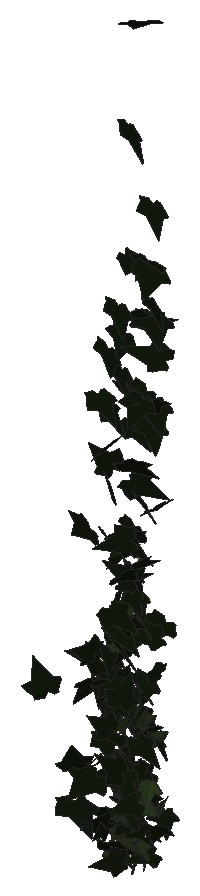
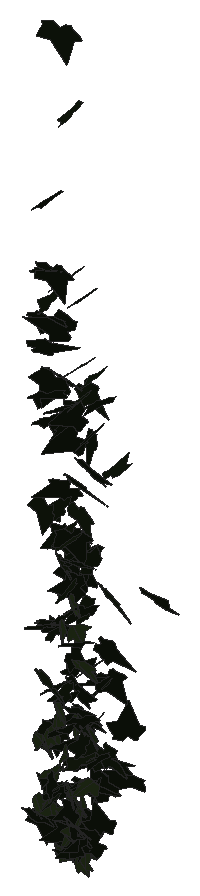
# SketchUp Ruby script. Lengths in inches.
U = 1.inch
M = Sketchup.active_model
def pt(a) = Geom::Point3d.new(a.map { |v| v * U })
def face(e, loops, mat)
  f = e.add_face(loops[0].map { |a| pt(a) })
  loops[1..].each { |l| e.add_face(l.map { |a| pt(a) }).erase! }
  f.material = f.back_material = mat if mat
  f
end
# faces: each face lists its corners as indices into pts; further lists are holes
def faces(e, pts, list, mat = nil) = list.each { |f| face(e, (f[0].is_a?(Array) ? f : [f]).map { |l| l.map { |i| pts[i] } }, mat) }
# xy, xz, yz: faces in a plane at the given z, y or x. An outline is a flat list of corners, or four numbers for a rectangle; further outlines are holes
def ring(l) = l.size == 4 ? [[l[0], l[1]], [l[2], l[1]], [l[2], l[3]], [l[0], l[3]]] : l.each_slice(2).to_a
def flat(e, list, mat, &to3) = list.each { |f| face(e, (f[0].is_a?(Array) ? f : [f]).map { |l| ring(l).map { |u, v| to3.(u, v) } }, mat) }
def xy(e, z, list, mat = nil) = flat(e, list, mat) { |x, y| [x, y, z] }
def xz(e, y, list, mat = nil) = flat(e, list, mat) { |x, z| [x, y, z] }
def yz(e, x, list, mat = nil) = flat(e, list, mat) { |y, z| [x, y, z] }
def lines(e, pts, list) = list.each { |a, b| e.add_line(pt(pts[a]), pt(pts[b])) }
# prism: a flat outline (further loops are holes) pulled along v
def prism(e, loops, v, mat = nil)
  f = face(e, loops, mat); d = Geom::Vector3d.new(v.map { |x| x * U })
  f.pushpull(f.normal.samedirection?(d) ? d.length : -d.length)
end
def box(e, o, s, mat = nil) = prism(e, [[o, [o[0] + s[0], o[1], o[2]], [o[0] + s[0], o[1] + s[1], o[2]], [o[0], o[1] + s[1], o[2]]]], [0, 0, s[2]], mat)
def at(x, y, z, deg = 0) = Geom::Transformation.translation(pt([x, y, z])) * Geom::Transformation.rotation(ORIGIN, Z_AXIS, deg.degrees)
def axes(o, x, y, z) = Geom::Transformation.new([*x, 0, *y, 0, *z, 0, *pt(o).to_a, 1])
def part(name) = M.definitions.add(name)
# library, detail: a bought-in or finely detailed component or shape, given as its bounding box
def library(name, o, s) = part(name).tap { |d| box(d.entities, o, s) }
def detail(e, o, s) = box(e.add_group.entities, o, s)
def put(e, d, t, mat = nil) = e.add_instance(d, t).tap { |i| i.material = mat if mat }
def group(e, t, mat = nil) = e.add_group.tap { |g| g.transformation = t; g.material = mat if mat }.entities
root = M.entities
M.materials.add("1026 AP 7946 SUNNY SIDE UP").color = [254, 231, 186]
M.materials.add("efeu1").color = [18, 25, 13]
M.materials.add("efeu2").color = [43, 57, 29]
c1 = part("ivyleaf_10")
p = [[0,0.5,-0.03],[-0.0625,2.02,-0.43],[-0.19,2.01,-0.46],[-0.54,1.05,-0.29],[-0.52,0.625,-0.18],[-0.83,0.76,-0.28],
  [-1.16,0.64,-0.33],[-1.15,0.33,-0.24],[-0.77,-0.39,0.02],[-0.3,-0.51,0.16],[0.04,-0.48,0.23],[-0.02,2.01,-0.4375],
  [-0.06,2.01,-0.43],[0.04,-0.49,0.23],[0.67,-0.49,0.14],[1.38,0.36,-0.2],[1.375,0.51,-0.24],[0.81,0.65,-0.19],
  [0.62,0.59,-0.15],[0.6,1.09,-0.28],[0.5,1.23,-0.31]]
faces(c1.entities,p,[[0,1,2,3,4,5,6,7,8,9,10],[11,12,0,13,14,15,16,17,18,19,20]],"efeu2")
c2 = part("ivyleaf_9")
p = [[1.54,2.16,1.25],[1.36,2.04,1.19],[-0.21,0.99,0.68],[-0.71,1.11,0.82],[-0.85,0.86,0.67],[-0.8,0.17,0.21],
  [-0.9,-0.01,0.1],[-0.67,-0.16,-0.02],[-0.08,-0.08,-0.05],[-0.03,-0.6,-0.4],[0.65,-0.88,-0.66],[0.83,-0.6,-0.49],
  [1.29,-0.42,-0.43],[1.8125,-0.07,-0.26],[1.21,0.44,0.15]]
faces(c2.entities,p,[[0,1,2,3,4,5,6,7,8,9,10,11,12,13,14]],"efeu1")
put(root,c1,axes([137.83,211.51,297.38],[0.4012,-0.28176,-0.05488],[-0.07373,0.02718,-0.39107],[0.44435,0.25891,-0.01534]),"1026 AP 7946 SUNNY SIDE UP")
put(root,c2,axes([137.54,211.69,314.56],[0.01331,-0.40991,0.19079],[0.02943,-0.18708,-0.42325],[0.70819,0.01547,0.014]),"1026 AP 7946 SUNNY SIDE UP")
put(root,c2,axes([138.35,209.95,300.61],[-0.17209,0.02371,-0.4585],[-0.6701,-0.14021,0.09942],[-0.2059,0.43649,0.05967]),"1026 AP 7946 SUNNY SIDE UP")
put(root,c2,axes([137.45,211.55,292.13],[0.51397,0.13779,0.20311],[0.29466,0.06056,-0.36476],[-0.23551,0.37648,-0.01311]),"1026 AP 7946 SUNNY SIDE UP")
put(root,c2,axes([138.01,210.06,299.29],[-0.00822,0.28996,-0.33221],[0.02756,-0.32374,-0.30055],[-0.68326,-0.01655,-0.00812]),"1026 AP 7946 SUNNY SIDE UP")
put(root,c2,axes([137.67,211.26,296],[-0.00138,-0.36582,-0.11151],[-0.01405,0.10615,-0.37614],[0.59879,0.00165,-0.00908]),"1026 AP 7946 SUNNY SIDE UP")
put(root,c1,axes([137.91,212.06,291.31],[-0.03657,-0.34127,0.1456],[-0.00683,-0.14329,-0.35319],[0.58194,-0.02313,0.005]),"1026 AP 7946 SUNNY SIDE UP")
put(root,c2,axes([137.6,211.53,311.9],[0.26933,-0.37215,-0.18863],[-0.11711,0.16496,-0.42108],[0.64008,0.18677,0.00233]),"1026 AP 7946 SUNNY SIDE UP")
put(root,c1,axes([138.09,211.77,291.07],[-0.4496,0.1913,-0.15349],[-0.17696,0.10123,0.35442],[0.3389,0.30664,-0.01857]),"1026 AP 7946 SUNNY SIDE UP")
put(root,c2,axes([137.67,211.29,297.84],[0.3313,-0.2889,-0.23528],[-0.14859,0.20996,-0.36483],[0.55803,0.22743,0.04254]),"1026 AP 7946 SUNNY SIDE UP")
put(root,c2,axes([138.39,210.875,309.48],[-0.09102,0.24213,0.41038],[-0.42897,0.30627,-0.23164],[-0.5921,-0.25911,0.10473]),"1026 AP 7946 SUNNY SIDE UP")
put(root,c1,axes([137.73,211.64,294.87],[-0.22919,-0.20056,-0.30427],[0.34422,0.20026,-0.25118],[0.44157,-0.2602,0.03788]),"1026 AP 7946 SUNNY SIDE UP")
put(root,c2,axes([138.15,210.05,295.625],[-0.32693,0.29532,-0.22341],[0.12696,-0.20824,-0.37025],[-0.56356,-0.21823,0.04619]),"1026 AP 7946 SUNNY SIDE UP")
put(root,c2,axes([137.67,210.85,292.39],[0.61428,-0.06207,-0.01055],[0.02521,0.03823,0.40561],[-0.09556,-0.38891,0.0392]),"1026 AP 7946 SUNNY SIDE UP")
put(root,c1,axes([138.18,211.67,300.53],[0.49868,-0.12912,-0.19854],[-0.30965,0.02036,-0.34911],[0.19098,0.37017,-0.04761]),"1026 AP 7946 SUNNY SIDE UP")
put(root,c2,axes([137.94,211.94,298.11],[-0.20399,-0.34986,-0.10126],[0.05213,0.09042,-0.38387],[0.56819,-0.1339,-0.00113]),"1026 AP 7946 SUNNY SIDE UP")
put(root,c2,axes([137.95,212.26,315.18],[-0.14688,-0.37961,0.20878],[-0.00701,-0.2087,-0.40181],[0.6782,-0.08437,0.04106]),"1026 AP 7946 SUNNY SIDE UP")
put(root,c2,axes([137.68,211.54,305.46],[0.1914,-0.26591,0.33434],[0.23774,-0.2891,-0.30273],[0.61737,0.19377,0.01293]),"1026 AP 7946 SUNNY SIDE UP")
put(root,c2,axes([137.72,212.07,296.91],[0.37537,-0.28468,0.14955],[0.10506,-0.13478,-0.38203],[0.49256,0.2457,-0.03249]),"1026 AP 7946 SUNNY SIDE UP")
put(root,c2,axes([138.34,209.76,294.98],[-0.6747,-0.20928,0.03821],[-0.02552,-0.05372,-0.49032],[0.33356,-0.42743,0.03977]),"1026 AP 7946 SUNNY SIDE UP")
put(root,c2,axes([138.07,208.66,295.9],[0.43434,0.21469,0.30903],[-0.40918,-0.15006,0.35808],[0.40892,-0.3782,0.03007]),"1026 AP 7946 SUNNY SIDE UP")
put(root,c2,axes([138.65,211.18,294.4],[-0.5417,0.0012,0.27766],[-0.42114,-0.05037,-0.35275],[0.04732,-0.43449,0.03909]),"1026 AP 7946 SUNNY SIDE UP")
put(root,c2,axes([137.9,210.63,312.9],[0.09758,-0.39034,-0.19905],[0.02644,0.19495,-0.40368],[0.6828,0.04824,0.04407]),"1026 AP 7946 SUNNY SIDE UP")
put(root,c2,axes([137.96,212.09,313.51],[0.08002,-0.41551,0.10142],[-0.00389,-0.1018,-0.43159],[0.67229,0.04887,-0.01457]),"1026 AP 7946 SUNNY SIDE UP")
put(root,c2,axes([138.04,210.51,298.89],[-0.02751,-0.31744,0.23075],[0.00706,-0.22617,-0.32854],[0.61249,-0.01165,0.01415]),"1026 AP 7946 SUNNY SIDE UP")
put(root,c1,axes([138.29,211.92,302.27],[-0.24082,-0.31947,0.17507],[0.06064,-0.19973,-0.34845],[0.5671,-0.11431,0.11161]),"1026 AP 7946 SUNNY SIDE UP")
put(root,c2,axes([138.09,211.24,300.18],[-0.05447,-0.38917,0.11404],[-0.00962,-0.11281,-0.40315],[0.6371,-0.03498,0.00366]),"1026 AP 7946 SUNNY SIDE UP")
put(root,c2,axes([138,208.9,293.96],[-0.29707,-0.26418,-0.36455],[0.39707,0.24915,-0.33046],[0.56735,-0.3127,0.0404]),"1026 AP 7946 SUNNY SIDE UP")
put(root,c2,axes([138.73,211.28,298.89],[-0.06949,0.10664,0.46598],[-0.3435,0.39558,-0.11591],[-0.64392,-0.22253,0.01154]),"1026 AP 7946 SUNNY SIDE UP")
put(root,c1,axes([138.32,211.61,293.21],[-0.3447,0.29579,0.03313],[-0.06057,0.00929,-0.37833],[-0.46362,-0.22113,0.0248]),"1026 AP 7946 SUNNY SIDE UP")
put(root,c2,axes([138.375,212.02,294.69],[-0.25939,-0.21116,0.2866],[-0.17091,-0.26272,-0.27221],[0.52349,-0.19041,0.05314]),"1026 AP 7946 SUNNY SIDE UP")
put(root,c2,axes([138.29,212.125,301.71],[-0.34152,-0.32796,0.04261],[0.07011,-0.08026,-0.39702],[0.51539,-0.2064,0.08224]),"1026 AP 7946 SUNNY SIDE UP")
put(root,c2,axes([138.76,206.01,300.99],[-0.71849,0.06801,-0.137],[-0.20114,0.04522,0.47549],[0.12232,0.47385,-0.02285]),"1026 AP 7946 SUNNY SIDE UP")
put(root,c2,axes([138.39,211,299.3125],[-0.33496,-0.33533,0.14859],[-0.07402,-0.14257,-0.40856],[0.57038,-0.21542,0.03424]),"1026 AP 7946 SUNNY SIDE UP")
put(root,c2,axes([137.96,212.05,312.84],[0.65535,-0.11657,0.09573],[0.12224,-0.06776,-0.444],[0.20077,0.42175,-0.04216]),"1026 AP 7946 SUNNY SIDE UP")
put(root,c2,axes([138.02,211.89,295.85],[0.05295,-0.43187,0.13889],[0.24199,-0.11857,-0.42388],[0.67019,0.07693,0.14208]),"1026 AP 7946 SUNNY SIDE UP")
put(root,c2,axes([138.52,211.8125,305.46],[-0.57268,-0.16871,-0.04043],[0.12797,-0.08835,-0.39703],[0.24004,-0.3554,0.11522]),"1026 AP 7946 SUNNY SIDE UP")
put(root,c2,axes([138.48,211.31,297.53],[-0.38477,0.14602,-0.29034],[0.34675,-0.17918,-0.29309],[-0.36058,-0.32813,0.02797]),"1026 AP 7946 SUNNY SIDE UP")
put(root,c2,axes([138.1,211.93,291.69],[0.50683,-0.17534,0.05451],[0.04919,-0.05485,-0.37681],[0.28421,0.32217,-0.03199]),"1026 AP 7946 SUNNY SIDE UP")
put(root,c2,axes([138.31,210.33,295.53],[-0.09367,0.39647,-0.18602],[-0.03098,0.18188,0.41403],[0.6858,0.06237,-0.00671]),"1026 AP 7946 SUNNY SIDE UP")
put(root,c2,axes([138.91,211.92,292.9375],[-0.36654,0.22115,0.20028],[-0.27084,0.09674,-0.32769],[-0.37391,-0.28686,0.04103]),"1026 AP 7946 SUNNY SIDE UP")
put(root,c1,axes([138.62,211.98,294.51],[0.20419,-0.30117,-0.21215],[-0.1395,0.18408,-0.33672],[0.5549,0.15711,-0.00659]),"1026 AP 7946 SUNNY SIDE UP")
put(root,c2,axes([138.01,211.98,291.92],[0.4199,-0.14774,0.26811],[0.33213,-0.15562,-0.31419],[0.33495,0.33951,-0.02456]),"1026 AP 7946 SUNNY SIDE UP")
put(root,c2,axes([138.6,211.48,291.7],[-0.40329,0.29124,-0.04141],[-0.02237,0.04317,0.39963],[0.46211,0.25626,-0.01679]),"1026 AP 7946 SUNNY SIDE UP")
put(root,c2,axes([138.82,211.33,297.99],[-0.61747,-0.07745,0.04565],[-0.05714,-0.04596,-0.41077],[0.12852,-0.39255,0.03667]),"1026 AP 7946 SUNNY SIDE UP")
put(root,c1,axes([138.42,211.7,292.39],[-0.36047,-0.24316,-0.20815],[0.27678,0.10712,-0.34026],[0.41127,-0.28521,0.04655]),"1026 AP 7946 SUNNY SIDE UP")
put(root,c1,axes([138.55,211.8,303.49],[0.21611,-0.34974,0.13106],[0.05423,-0.12518,-0.38763],[0.58375,0.14111,-0.01251]),"1026 AP 7946 SUNNY SIDE UP")
put(root,c1,axes([139.03,211.3,293.49],[-0.16669,0.09849,0.35885],[-0.55507,0.04967,-0.12505],[-0.12213,-0.36017,0.07858]),"1026 AP 7946 SUNNY SIDE UP")
put(root,c2,axes([138.52,211.76,293.34],[0.1528,0.1864,0.32703],[0.2826,0.26126,-0.21391],[-0.50352,0.2032,-0.02082]),"1026 AP 7946 SUNNY SIDE UP")
put(root,c1,axes([138.625,212.3,296.36],[-0.02972,0.25303,-0.30258],[-0.0139,-0.2957,-0.2623],[-0.61113,-0.00558,0.02068]),"1026 AP 7946 SUNNY SIDE UP")
put(root,c2,axes([138.95,211.88,291.33],[-0.53508,-0.12315,0.05816],[-0.06758,-0.04858,-0.37176],[0.20249,-0.34162,0.0296]),"1026 AP 7946 SUNNY SIDE UP")
put(root,c1,axes([138.63,210.82,291.07],[-0.3755,-0.21027,-0.17548],[0.28174,0.04534,-0.31841],[0.31729,-0.28911,0.07507]),"1026 AP 7946 SUNNY SIDE UP")
put(root,c2,axes([138.82,211.48,300.74],[-0.15976,0.14562,-0.38123],[0.29349,-0.32077,-0.1843],[-0.55353,-0.2121,0.01231]),"1026 AP 7946 SUNNY SIDE UP")
put(root,c2,axes([138.5,211.79,319.36],[0.35909,-0.33894,-0.22388],[-0.08184,0.22071,-0.41336],[0.62613,0.22324,0.07436]),"1026 AP 7946 SUNNY SIDE UP")
put(root,c2,axes([138.73,212.0625,297.45],[-0.17677,-0.36124,0.04195],[-0.00377,-0.04403,-0.38986],[0.57197,-0.11194,0.01039]),"1026 AP 7946 SUNNY SIDE UP")
put(root,c2,axes([139.03,211.24,306.33],[0.1522,0.33957,-0.27374],[-0.09624,-0.26075,-0.36513],[-0.67301,0.11408,-0.00969]),"1026 AP 7946 SUNNY SIDE UP")
put(root,c2,axes([138.33,211.85,292.28],[0.00097,-0.07821,-0.48898],[0.57512,0.3077,-0.04999],[0.49025,-0.36082,0.05961]),"1026 AP 7946 SUNNY SIDE UP")
put(root,c1,axes([138.89,210.75,293.28],[0.15458,-0.32954,-0.21242],[0.03113,0.21478,-0.34579],[0.60889,0.07268,0.07161]),"1026 AP 7946 SUNNY SIDE UP")
put(root,c2,axes([138.74,212.31,296.78],[-0.1279,-0.37344,0.00884],[0.00588,-0.01177,-0.39375],[0.58741,-0.0812,0.00587]),"1026 AP 7946 SUNNY SIDE UP")
put(root,c2,axes([138.58,212.09,304.07],[0.16065,-0.3766,0.15164],[0.04144,-0.1475,-0.40266],[0.63567,0.10479,-0.01207]),"1026 AP 7946 SUNNY SIDE UP")
put(root,c2,axes([138.6875,212.1,302.96],[0.05258,-0.42335,-0.05714],[-0.02251,0.05208,-0.43706],[0.6705,0.03495,-0.01019]),"1026 AP 7946 SUNNY SIDE UP")
put(root,c2,axes([138.75,211.93,306.28],[-0.1103,-0.3326,0.23208],[0.04421,-0.23407,-0.34547],[0.63178,-0.04169,0.0647]),"1026 AP 7946 SUNNY SIDE UP")
put(root,c1,axes([138.94,210.96,297.31],[-0.01767,-0.37872,-0.14308],[0.06137,0.13512,-0.38806],[0.63014,-0.02378,0.03378]),"1026 AP 7946 SUNNY SIDE UP")
put(root,c2,axes([138.68,211.22,303.88],[0.20812,0.15279,0.39844],[0.45912,0.25358,-0.20512],[-0.4638,0.31958,-0.02426]),"1026 AP 7946 SUNNY SIDE UP")
put(root,c2,axes([139.21,211.82,330.98],[0.22632,0.44363,-0.10633],[-0.23462,-0.05896,-0.46446],[-0.67764,0.16858,0.1253]),"1026 AP 7946 SUNNY SIDE UP")
put(root,c1,axes([138.85,211.43,291.28],[-0.46663,-0.16687,-0.15755],[0.26352,0.00526,-0.34304],[0.23773,-0.33338,0.07101]),"1026 AP 7946 SUNNY SIDE UP")
put(root,c1,axes([139.04,211.95,302.37],[0.35366,-0.31054,-0.10888],[0.0137,0.13171,-0.38524],[0.51472,0.20986,0.08507]),"1026 AP 7946 SUNNY SIDE UP")
put(root,c2,axes([138.86,211.55,292.92],[-0.05808,-0.37097,-0.08603],[0.04003,0.07919,-0.38319],[0.59585,-0.04148,0.01736]),"1026 AP 7946 SUNNY SIDE UP")
put(root,c2,axes([139.5,208.26,302.0625],[-0.37994,0.35783,0.17823],[-0.17097,0.13276,-0.44378],[-0.59969,-0.26456,0.0136]),"1026 AP 7946 SUNNY SIDE UP")
put(root,c2,axes([139.09,212.27,312.8125],[-0.35496,-0.32314,0.17721],[-0.05067,-0.18587,-0.4001],[0.57474,-0.21595,0.07417]),"1026 AP 7946 SUNNY SIDE UP")
put(root,c2,axes([138.82,209.08,292.97],[0.49659,0.29216,0.10893],[-0.15698,-0.04487,0.44158],[0.46172,-0.32948,0.03297]),"1026 AP 7946 SUNNY SIDE UP")
put(root,c2,axes([138.75,211.84,299.03],[0.43938,-0.27258,0.02814],[0.00719,-0.03657,-0.40167],[0.43095,0.27853,-0.02199]),"1026 AP 7946 SUNNY SIDE UP")
put(root,c2,axes([139.02,211.6,298.68],[-0.19779,-0.36412,0.05604],[-0.00849,-0.05784,-0.39695],[0.57932,-0.12516,0.01332]),"1026 AP 7946 SUNNY SIDE UP")
put(root,c2,axes([138.94,212.04,297.3],[0.19255,-0.27874,-0.26677],[-0.0578,0.26046,-0.30709],[0.59374,0.11575,0.05662]),"1026 AP 7946 SUNNY SIDE UP")
put(root,c2,axes([138.94,210.62,317.5625],[0.0218,-0.44722,0.06102],[0.00222,-0.06176,-0.46131],[0.70988,0.01393,-0.00043]),"1026 AP 7946 SUNNY SIDE UP")
put(root,c2,axes([139.16,208.3125,307.95],[-0.36413,-0.18579,0.38399],[-0.01767,-0.42453,-0.22704],[0.65611,-0.11454,0.20699]),"1026 AP 7946 SUNNY SIDE UP")
put(root,c2,axes([139.58,210.65,294.71],[-0.33883,-0.05141,0.36616],[-0.4782,-0.19495,-0.21996],[0.30117,-0.36737,0.06269]),"1026 AP 7946 SUNNY SIDE UP")
put(root,c2,axes([139.3,209.95,303.39],[-0.0023,-0.01127,0.48334],[0.22189,0.44753,0.01414],[-0.70391,0.14111,0.00288]),"1026 AP 7946 SUNNY SIDE UP")
put(root,c2,axes([139.27,212.32,294.35],[-0.28665,-0.19834,0.26709],[-0.07785,-0.27791,-0.25542],[0.50877,-0.15427,0.1114]),"1026 AP 7946 SUNNY SIDE UP")
put(root,c2,axes([139.46,211.98,319.32],[0.41668,0.11052,-0.36401],[-0.45368,-0.21184,-0.2919],[-0.36627,0.38812,-0.05254]),"1026 AP 7946 SUNNY SIDE UP")
put(root,c1,axes([139.31,211.81,298.11],[0.20049,-0.35804,0.06534],[0.00349,-0.06859,-0.39137],[0.57231,0.12585,-0.0205]),"1026 AP 7946 SUNNY SIDE UP")
put(root,c1,axes([139.36,212.27,297.04],[-0.06699,-0.34072,0.17404],[-0.00435,-0.17166,-0.35433],[0.59933,-0.03933,0.01688]),"1026 AP 7946 SUNNY SIDE UP")
put(root,c2,axes([139.17,209.47,293.06],[0.01214,-0.17579,-0.3825],[0.40772,-0.28474,0.14317],[-0.49918,-0.23685,0.10763]),"1026 AP 7946 SUNNY SIDE UP")
put(root,c2,axes([139.55,210.75,304.55],[-0.11146,-0.42847,-0.07252],[0.02402,-0.07129,0.44617],[-0.68173,0.06754,0.02758]),"1026 AP 7946 SUNNY SIDE UP")
put(root,c2,axes([139.12,209.86,291.91],[0.68847,0.15163,-0.04197],[-0.03778,-0.0571,-0.47533],[-0.24433,0.43609,-0.04475]),"1026 AP 7946 SUNNY SIDE UP")
put(root,c2,axes([139.15,211.27,311.78],[0.20729,-0.33826,-0.24531],[-0.10243,0.22779,-0.37218],[0.64058,0.14588,0.01987]),"1026 AP 7946 SUNNY SIDE UP")
put(root,c2,axes([139,211.85,307.93],[0.35471,-0.31868,0.1355],[0.08474,-0.12483,-0.40202],[0.53653,0.2304,-0.02608]),"1026 AP 7946 SUNNY SIDE UP")
put(root,c2,axes([139,211.54,308.74],[0.10421,-0.06688,-0.44828],[0.21872,0.42029,-0.0423],[0.65616,-0.12947,0.08529]),"1026 AP 7946 SUNNY SIDE UP")
put(root,c2,axes([139.14,210.28,302.27],[0.09651,-0.32575,-0.31102],[-0.00027,0.30291,-0.33704],[0.69639,0.04526,0.04297]),"1026 AP 7946 SUNNY SIDE UP")
put(root,c2,axes([139.35,212.35,294.71],[-0.16787,0.02966,-0.39415],[0.42658,-0.27528,-0.10154],[-0.42714,-0.28658,0.0535]),"1026 AP 7946 SUNNY SIDE UP")
put(root,c1,axes([139.45,211.6875,297.44],[0.0252,-0.35835,-0.16728],[0.058,0.16114,-0.36627],[0.61457,-0.00052,0.04142]),"1026 AP 7946 SUNNY SIDE UP")
put(root,c2,axes([139.61,211.25,304.86],[-0.51194,0.15603,-0.23223],[0.28341,-0.14368,-0.37003],[-0.32634,-0.36955,0.04295]),"1026 AP 7946 SUNNY SIDE UP")
put(root,c2,axes([139.57,209.17,309.93],[0.41552,-0.12619,-0.38683],[-0.5546,0.12863,-0.30007],[0.28119,0.44016,-0.0202]),"1026 AP 7946 SUNNY SIDE UP")
put(root,c2,axes([139.72,210.89,293.69],[-0.38067,-0.1997,0.23649],[-0.2566,-0.16407,-0.32372],[0.40538,-0.29139,0.01716]),"1026 AP 7946 SUNNY SIDE UP")
put(root,c2,axes([139.53,211.74,301.88],[-0.39013,-0.30953,0.02548],[0.00397,-0.0359,-0.40811],[0.48847,-0.24692,0.02366]),"1026 AP 7946 SUNNY SIDE UP")
put(root,c2,axes([138.99,211.74,316.4375],[0.2598,-0.01027,0.43718],[0.6627,0.05887,-0.16721],[-0.08047,0.45163,0.03442]),"1026 AP 7946 SUNNY SIDE UP")
put(root,c2,axes([140,208.66,298.3],[-0.23921,0.28838,0.31781],[-0.28098,0.25122,-0.33302],[-0.59956,-0.23279,0.02927]),"1026 AP 7946 SUNNY SIDE UP")
put(root,c2,axes([139.47,211.96,299.09],[-0.16286,-0.36526,0.10704],[-0.02165,-0.10616,-0.39143],[0.59762,-0.10338,0.01499]),"1026 AP 7946 SUNNY SIDE UP")
put(root,c2,axes([139.31,212.22,293.74],[0.1746,-0.35718,0.05665],[0.01302,-0.05712,-0.38556],[0.56859,0.11099,-0.00856]),"1026 AP 7946 SUNNY SIDE UP")
put(root,c2,axes([139.71,211.56,296.87],[0.09526,0.38467,-0.02651],[0.00016,-0.02828,-0.40131],[-0.60644,0.06042,-0.00427]),"1026 AP 7946 SUNNY SIDE UP")
put(root,c2,axes([139.39,211.57,295.02],[0.32048,-0.29586,-0.22651],[-0.1766,0.18743,-0.36882],[0.5504,0.23241,0.01355]),"1026 AP 7946 SUNNY SIDE UP")
put(root,c2,axes([139.36,210.9,306.29],[0.44552,-0.2517,-0.1982],[-0.15373,0.17407,-0.38478],[0.4724,0.29402,0.06171]),"1026 AP 7946 SUNNY SIDE UP")
put(root,c2,axes([139.34,211.95,301.77],[0.02295,-0.2427,0.34221],[0.12796,-0.32551,-0.24957],[0.63589,0.07426,0.03787]),"1026 AP 7946 SUNNY SIDE UP")
put(root,c2,axes([140.02,212.02,299.56],[-0.40524,0.31206,0.01485],[-0.03613,-0.00259,-0.41648],[-0.48976,-0.25802,0.01844]),"1026 AP 7946 SUNNY SIDE UP")
put(root,c2,axes([139.69,209.89,298.95],[-0.36783,-0.12951,0.37647],[0.47537,0.20764,0.27584],[-0.3834,0.38169,-0.01917]),"1026 AP 7946 SUNNY SIDE UP")
put(root,c1,axes([139.67,211.79,292.92],[0.36325,0.27794,-0.12196],[0.08846,0.10886,0.37207],[0.46772,-0.23645,0.02435]),"1026 AP 7946 SUNNY SIDE UP")
put(root,c2,axes([140,209.09,312.13],[-0.31633,0.35267,-0.23962],[0.11241,-0.22772,-0.41715],[-0.65648,-0.20893,0.04404]),"1026 AP 7946 SUNNY SIDE UP")
put(root,c1,axes([139.6875,212.16,296.32],[0.31075,-0.30749,0.15822],[0.0955,-0.14517,-0.37651],[0.5332,0.2052,-0.02477]),"1026 AP 7946 SUNNY SIDE UP")
put(root,c2,axes([139.42,210.76,326.35],[0.24931,-0.45022,0.05772],[-0.00123,-0.06233,-0.49161],[0.71389,0.15712,-0.021]),"1026 AP 7946 SUNNY SIDE UP")
put(root,c2,axes([140.08,209.43,306.34],[-0.15235,0.43998,0.10264],[-0.06672,0.09,-0.46307],[-0.70534,-0.10355,0.02164]),"1026 AP 7946 SUNNY SIDE UP")
put(root,c2,axes([139.35,209.84,301.93],[0.44082,-0.35496,0.11262],[0.07481,-0.10406,-0.46579],[0.58016,0.28313,-0.02552]),"1026 AP 7946 SUNNY SIDE UP")
put(root,c2,axes([139.76,211.94,319.125],[-0.51887,-0.29241,-0.11942],[0.19222,0.03301,-0.45053],[0.45468,-0.34765,0.05418]),"1026 AP 7946 SUNNY SIDE UP")
put(root,c2,axes([139.92,211.82,307.64],[0.15163,0.40658,0.12242],[0.01038,0.11805,-0.42929],[-0.66496,0.09456,0.02122]),"1026 AP 7946 SUNNY SIDE UP")
put(root,c2,axes([139.8,209.76,305.2],[0.27457,0.38408,0.1743],[0.14077,0.14253,-0.43328],[-0.64333,0.19511,-0.02042]),"1026 AP 7946 SUNNY SIDE UP")
put(root,c2,axes([140.39,208.97,296.24],[-0.41192,0.00654,-0.39134],[-0.59706,0.01229,0.27003],[0.02174,0.46131,0.00106]),"1026 AP 7946 SUNNY SIDE UP")
put(root,c2,axes([139.5,211.72,293.71],[0.01104,-0.10957,0.37484],[0.37213,-0.28423,-0.09438],[0.46867,0.22826,0.06611]),"1026 AP 7946 SUNNY SIDE UP")
put(root,c1,axes([139.95,210.42,291.18],[0.09761,-0.16766,-0.37326],[-0.00827,0.36535,-0.17342],[0.62634,0.03095,0.05588]),"1026 AP 7946 SUNNY SIDE UP")
put(root,c2,axes([140.24,210.68,292.46],[-0.29693,0.30947,0.05752],[-0.08687,0.02939,-0.3719],[-0.48629,-0.19422,0.03131]),"1026 AP 7946 SUNNY SIDE UP")
put(root,c2,axes([140.39,209.01,291.91],[-0.58444,0.22444,0.08451],[-0.14865,-0.00133,-0.44444],[-0.34435,-0.38036,0.04843]),"1026 AP 7946 SUNNY SIDE UP")
put(root,c2,axes([140.49,211.7,315.08],[-0.32689,0.05404,0.41395],[-0.63125,-0.08815,-0.20243],[0.08564,-0.44346,0.08795]),"1026 AP 7946 SUNNY SIDE UP")
put(root,c2,axes([140.375,211.48,301.72],[-0.49613,-0.00333,0.24989],[-0.3507,-0.15263,-0.3019],[0.15012,-0.36757,0.12057]),"1026 AP 7946 SUNNY SIDE UP")
put(root,c2,axes([139.8125,211.9,316.84],[-0.41312,-0.24084,-0.29061],[0.36158,0.16335,-0.36513],[0.45554,-0.34807,0.02626]),"1026 AP 7946 SUNNY SIDE UP")
put(root,c1,axes([140.09,212.14,296.57],[-0.06609,-0.32827,0.20035],[-0.02712,-0.1957,-0.34202],[0.60085,-0.04494,0.0066]),"1026 AP 7946 SUNNY SIDE UP")
put(root,c2,axes([139.69,210.24,310.39],[0.62276,0.19672,0.1465],[0.20502,0.0546,-0.45517],[-0.32072,0.41688,-0.0065]),"1026 AP 7946 SUNNY SIDE UP")
put(root,c1,axes([140.11,210.98,291.19],[0.25002,-0.2685,-0.24312],[-0.07299,0.23895,-0.31294],[0.55574,0.15218,0.06827]),"1026 AP 7946 SUNNY SIDE UP")
put(root,c2,axes([140.01,209.49,303.4],[0.5667,0.21613,-0.1747],[-0.20825,-0.11068,-0.43282],[-0.37981,0.38316,-0.02335]),"1026 AP 7946 SUNNY SIDE UP")
put(root,c2,axes([140.4,210.63,291.84],[-0.25755,0.04169,-0.398],[-0.52826,0.196,0.16956],[0.30777,0.37129,-0.04202]),"1026 AP 7946 SUNNY SIDE UP")
put(root,c2,axes([139.72,211.85,317.61],[0.20738,-0.39863,0.16521],[0.05772,-0.15906,-0.43325],[0.6745,0.13618,-0.01372]),"1026 AP 7946 SUNNY SIDE UP")
put(root,c2,axes([140.11,212.28,301.96],[-0.42405,-0.27821,0.12056],[-0.01056,-0.15337,-0.38722],[0.47543,-0.25154,0.09893]),"1026 AP 7946 SUNNY SIDE UP")
put(root,c2,axes([140.16,211.48,292.4],[0.38986,0.24257,-0.17834],[-0.17726,-0.13405,-0.35778],[-0.43513,0.27194,-0.01404]),"1026 AP 7946 SUNNY SIDE UP")
put(root,c2,axes([139.79,212.06,296.49],[0.1833,-0.33099,0.15137],[0.0817,-0.13947,-0.36233],[0.56476,0.12761,0.00329]),"1026 AP 7946 SUNNY SIDE UP")
put(root,c2,axes([139.97,211.625,311.84],[-0.11671,-0.41342,-0.05997],[0.0282,0.05352,-0.43231],[0.65536,-0.07592,0.00793]),"1026 AP 7946 SUNNY SIDE UP")
put(root,c1,axes([140.11,211.21,294.53],[0.24343,0.337,-0.15506],[-0.06853,-0.14747,-0.38235],[-0.57754,0.15954,-0.01999]),"1026 AP 7946 SUNNY SIDE UP")
put(root,c2,axes([140.16,210.7,313.43],[-0.59901,-0.12556,-0.21509],[0.36896,-0.08933,-0.38756],[0.09947,-0.42478,0.14227]),"1026 AP 7946 SUNNY SIDE UP")
put(root,c1,axes([139.99,210.49,292.03],[-0.48383,0.0288,-0.20329],[0.29473,-0.08297,-0.3138],[-0.1078,-0.35609,0.05446]),"1026 AP 7946 SUNNY SIDE UP")
put(root,c2,axes([140.03,210.375,305.46],[0.28382,0.21907,0.33137],[0.28176,0.26642,-0.29009],[-0.54139,0.25351,0.02275]),"1026 AP 7946 SUNNY SIDE UP")
put(root,c2,axes([139.99,211.66,322.41],[0.0182,-0.47044,0.00753],[-0.01789,-0.01027,-0.48471],[0.73968,0.01133,-0.01191]),"1026 AP 7946 SUNNY SIDE UP")
put(root,c1,axes([140.27,212.02,293.4],[0.03618,-0.37229,0.01773],[-0.00201,-0.01944,-0.38437],[0.58617,0.02291,-0.00241]),"1026 AP 7946 SUNNY SIDE UP")
put(root,c2,axes([140.72,209.16,307.5],[-0.67572,0.18228,0.09567],[-0.15906,-0.00431,-0.47891],[-0.27874,-0.43942,0.04137]),"1026 AP 7946 SUNNY SIDE UP")
put(root,c2,axes([140.01,210.67,296.9],[0.14722,-0.32311,-0.26908],[-0.01703,0.2639,-0.34117],[0.65127,0.07994,0.0519]),"1026 AP 7946 SUNNY SIDE UP")
put(root,c2,axes([140.08,211.55,312.91],[-0.16874,-0.39902,-0.19088],[0.11334,0.16984,-0.424],[0.6809,-0.12716,0.02327]),"1026 AP 7946 SUNNY SIDE UP")
put(root,c2,axes([140.3,210.83,313.25],[0.39419,0.37455,0.01375],[0.03981,-0.00347,-0.46373],[-0.58787,0.25092,-0.02219]),"1026 AP 7946 SUNNY SIDE UP")
put(root,c2,axes([140.17,212.17,292.82],[-0.34227,-0.16984,-0.24681],[0.39385,0.04613,-0.26896],[0.23868,-0.31967,0.08988]),"1026 AP 7946 SUNNY SIDE UP")
put(root,c2,axes([140.15,208.68,304.16],[0.09228,-0.23284,-0.42717],[-0.07171,0.41178,-0.24324],[0.7425,0.06871,0.0296]),"1026 AP 7946 SUNNY SIDE UP")
put(root,c2,axes([140.57,210.9,291.53],[-0.41278,-0.15633,0.22542],[-0.19974,-0.19876,-0.30324],[0.37399,-0.2787,0.08685]),"1026 AP 7946 SUNNY SIDE UP")
